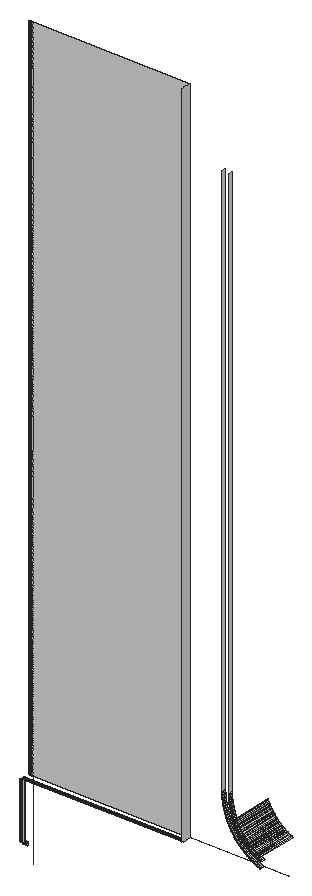
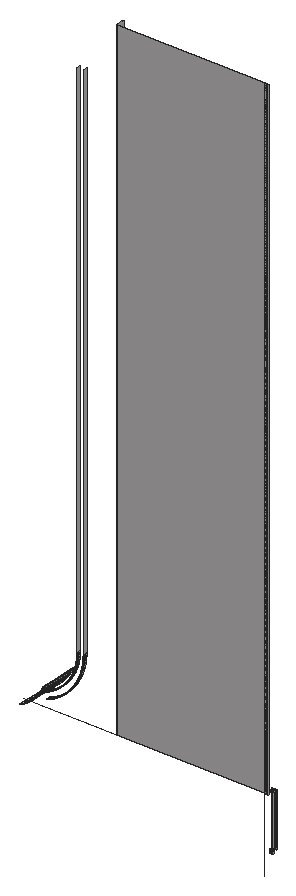
# SketchUp Ruby script. Lengths in inches.
U = 1.inch
M = Sketchup.active_model
def pt(a) = Geom::Point3d.new(a.map { |v| v * U })
def face(e, loops, mat)
  f = e.add_face(loops[0].map { |a| pt(a) })
  loops[1..].each { |l| e.add_face(l.map { |a| pt(a) }).erase! }
  f.material = f.back_material = mat if mat
  f
end
# faces: each face lists its corners as indices into pts; further lists are holes
def faces(e, pts, list, mat = nil) = list.each { |f| face(e, (f[0].is_a?(Array) ? f : [f]).map { |l| l.map { |i| pts[i] } }, mat) }
# xy, xz, yz: faces in a plane at the given z, y or x. An outline is a flat list of corners, or four numbers for a rectangle; further outlines are holes
def ring(l) = l.size == 4 ? [[l[0], l[1]], [l[2], l[1]], [l[2], l[3]], [l[0], l[3]]] : l.each_slice(2).to_a
def flat(e, list, mat, &to3) = list.each { |f| face(e, (f[0].is_a?(Array) ? f : [f]).map { |l| ring(l).map { |u, v| to3.(u, v) } }, mat) }
def xy(e, z, list, mat = nil) = flat(e, list, mat) { |x, y| [x, y, z] }
def xz(e, y, list, mat = nil) = flat(e, list, mat) { |x, z| [x, y, z] }
def yz(e, x, list, mat = nil) = flat(e, list, mat) { |y, z| [x, y, z] }
def lines(e, pts, list) = list.each { |a, b| e.add_line(pt(pts[a]), pt(pts[b])) }
# prism: a flat outline (further loops are holes) pulled along v
def prism(e, loops, v, mat = nil)
  f = face(e, loops, mat); d = Geom::Vector3d.new(v.map { |x| x * U })
  f.pushpull(f.normal.samedirection?(d) ? d.length : -d.length)
end
def box(e, o, s, mat = nil) = prism(e, [[o, [o[0] + s[0], o[1], o[2]], [o[0] + s[0], o[1] + s[1], o[2]], [o[0], o[1] + s[1], o[2]]]], [0, 0, s[2]], mat)
def at(x, y, z, deg = 0) = Geom::Transformation.translation(pt([x, y, z])) * Geom::Transformation.rotation(ORIGIN, Z_AXIS, deg.degrees)
def axes(o, x, y, z) = Geom::Transformation.new([*x, 0, *y, 0, *z, 0, *pt(o).to_a, 1])
def part(name) = M.definitions.add(name)
# library, detail: a bought-in or finely detailed component or shape, given as its bounding box
def library(name, o, s) = part(name).tap { |d| box(d.entities, o, s) }
def detail(e, o, s) = box(e.add_group.entities, o, s)
def put(e, d, t, mat = nil) = e.add_instance(d, t).tap { |i| i.material = mat if mat }
def group(e, t, mat = nil) = e.add_group.tap { |g| g.transformation = t; g.material = mat if mat }.entities
root = M.entities
M.materials.add("[Quartz Light Brown]").color = [215, 212, 212]
xz(root,143,[[215.8,133,216,150]],"[Quartz Light Brown]")
xz(root,143.01,[[215.41,133,215.61,150]],"[Quartz Light Brown]")
xz(root,143.75,[[215.625,149.75,215.8125,150],[215.8125,149.75,216,150],[216,149.75,263.5,150]],"[Quartz Light Brown]")
xz(root,144,[[215.63,132,215.82,133],[215.82,132,216,133]],"[Quartz Light Brown]")
xz(root,144.25,[[215.64,149.75,215.82,150],[215.82,149.75,216,150],[216,149.75,263.5,150]],"[Quartz Light Brown]")
xz(root,146,[[215.6875,150,215.84,354],[215.84,150,216,354],[216,150,263.5,354]],"[Quartz Light Brown]")
yz(root,263.5,[[143.75,149.75,143.75,150,143,150,143,354,143.75,354,143.75,354.25,144.25,354.25,144.25,354,146,354,146,150,144.25,150,144.25,149.75]],"[Quartz Light Brown]")
yz(root,275.5,[[143,167.76,144.25,168],[143,168,144.25,336]],"[Quartz Light Brown]")
yz(root,275.51,[[143,167.29,144.25,167.53]],"[Quartz Light Brown]")
yz(root,277.5,[[143,167.79,144.25,168],[143,168,144.25,336]],"[Quartz Light Brown]")
yz(root,277.51,[[143,167.37,144.25,167.58]],"[Quartz Light Brown]")
p = [[214.72,144.06,133],[214.72,144.06,132],[214.9,144.04,132],[214.9,144.04,133],[215.08,144.03,132],[215.08,144.03,133],
  [215.27,144.02,132],[215.27,144.02,133],[215.45,144.01,132],[215.45,144.01,133],[215.63,144,132],[215.63,144,133],
  [214.54,144.08,133],[214.54,144.08,132],[214.82,143.05,133],[214.82,143.05,150],[214.63,143.0625,150],[214.63,143.0625,133],
  [215.02,143.03,133],[215.02,143.03,150],[215.21,143.02,133],[215.21,143.02,150],[215.41,143.01,133],[215.41,143.01,150],
  [215.8,143,133],[215.8,143,150],[215.61,143.01,150],[215.61,143.01,133],[214.43,143.08,150],[214.43,143.08,133],
  [214.51,143.83,150],[214.7,143.81,150],[214.7,143.81,149.75],[214.51,143.83,149.75],[214.88,143.79,150],[214.88,143.79,149.75],
  [215.07,143.78,150],[215.07,143.78,149.75],[215.25,143.77,150],[215.25,143.77,149.75],[215.44,143.76,150],[215.44,143.76,149.75],
  [215.625,143.75,150],[215.625,143.75,149.75],[214.74,144.31,150],[214.5625,144.33,150],[214.5625,144.33,149.75],[214.74,144.31,149.75],
  [214.92,144.29,150],[214.92,144.29,149.75],[215.1,144.28,150],[215.1,144.28,149.75],[215.28,144.27,150],[215.28,144.27,149.75],
  [215.46,144.26,150],[215.46,144.26,149.75],[215.64,144.25,150],[215.64,144.25,149.75],[215.06,146.04,150],[215.06,146.04,354],
  [214.9,146.05,354],[214.9,146.05,150],[215.22,146.03,150],[215.22,146.03,354],[215.37,146.02,150],[215.37,146.02,354],
  [215.53,146.01,150],[215.53,146.01,354],[215.6875,146,150],[215.6875,146,354],[214.75,146.07,150],[214.75,146.07,354],
  [214.59,146.08,354],[214.59,146.08,150],[287.05,144.25,151.2],[287.05,143,151.2],[287.27,143,151.11],[287.27,144.25,151.11],
  [286.83,144.25,151.28],[286.83,143,151.28],[286.61,144.25,151.37],[286.61,143,151.37],[286.39,144.25,151.46],[286.39,143,151.46],
  [286.18,144.25,151.56],[286.18,143,151.56],[285.96,144.25,151.65],[285.96,143,151.65],[285.75,144.25,151.75],[285.75,143,151.75],
  [285.54,144.25,151.86],[285.54,143,151.86],[285.33,144.25,151.96],[285.33,143,151.96],[285.12,144.25,152.07],[285.12,143,152.07],
  [284.91,144.25,152.18],[284.91,143,152.18],[284.7,144.25,152.3],[284.7,143,152.3],[284.5,144.25,152.41],[284.5,143,152.41],
  [284.3,144.25,152.53],[284.3,143,152.53],[284.1,144.25,152.65],[284.1,143,152.65],[283.89,144.25,152.78],[283.89,143,152.78],
  [283.7,144.25,152.9],[283.7,143,152.9],[283.5,144.25,153.03],[283.5,143,153.03],[283.3,144.25,153.17],[283.3,143,153.17],
  [283.11,144.25,153.3],[283.11,143,153.3],[287.38,143,153.22],[287.18,143,153.3],[287.18,144.25,153.3],[287.38,144.25,153.22],
  [282.92,144.25,153.4375],[282.92,143,153.4375],[286.99,143,153.38],[286.99,144.25,153.38],[282.73,144.25,153.58],[282.73,143,153.58],
  [286.8,143,153.47],[286.8,144.25,153.47],[286.61,143,153.56],[286.61,144.25,153.56],[282.54,144.25,153.72],[282.54,143,153.72],
  [286.42,143,153.65],[286.42,144.25,153.65],[282.36,144.25,153.86],[282.36,143,153.86],[286.24,143,153.74],[286.05,143,153.84],
  [286.05,144.25,153.84],[286.24,144.25,153.74],[285.87,143,153.9375],[285.87,144.25,153.9375],[282.17,144.25,154.01],[282.17,143,154.01],
  [285.68,143,154.04],[285.68,144.25,154.04],[281.99,144.25,154.16],[281.99,143,154.16],[285.5,143,154.14],[285.5,144.25,154.14],
  [285.32,143,154.25],[285.32,144.25,154.25],[281.81,144.25,154.3125],[281.81,143,154.3125],[285.14,143,154.36],[285.14,144.25,154.36],
  [281.63,144.25,154.47],[281.63,143,154.47],[284.96,143,154.47],[284.96,144.25,154.47],[287.04,143,154.46],[287.22,143,154.38],
  [287.22,155,154.38],[287.04,155,154.46],[281.46,144.25,154.625],[281.46,143,154.625],[284.79,143,154.58],[284.79,144.25,154.58],
  [286.69,143,154.63],[286.87,143,154.55],[286.87,155,154.55],[286.69,155,154.63],[281.28,144.25,154.78],[281.28,143,154.78],
  [284.61,143,154.7],[284.61,144.25,154.7],[286.52,143,154.73],[286.52,155,154.73],[284.4375,143,154.8125],[284.4375,144.25,154.8125],
  [286.34,143,154.82],[286.34,155,154.82],[281.11,144.25,154.94],[281.11,143,154.94],[284.27,143,154.93],[284.27,144.25,154.93],
  [286.17,143,154.91],[286.17,155,154.91],[280.94,144.25,155.11],[280.94,143,155.11],[284.1,143,155.06],[284.1,144.25,155.06],
  [286,143,155.01],[286,155,155.01],[285.83,143,155.11],[285.83,155,155.11],[280.77,144.25,155.27],[280.77,143,155.27],
  [283.93,143,155.18],[283.93,144.25,155.18],[285.66,143,155.21],[285.66,155,155.21],[283.76,143,155.31],[283.76,144.25,155.31],
  [285.5,143,155.3125],[285.5,155,155.3125],[280.61,144.25,155.44],[280.61,143,155.44],[283.59,143,155.43],[283.59,144.25,155.43],
  [285.33,143,155.42],[285.33,155,155.42],[280.44,144.25,155.61],[280.44,143,155.61],[283.43,143,155.57],[283.43,144.25,155.57],
  [285.17,143,155.53],[285.17,155,155.53],[285,143,155.64],[285,155,155.64],[280.28,144.25,155.78],[280.28,143,155.78],
  [283.27,143,155.7],[283.27,144.25,155.7],[284.84,143,155.75],[284.84,155,155.75],[283.11,143,155.83],[283.11,144.25,155.83],
  [280.125,144.25,155.96],[280.125,143,155.96],[282.95,143,155.97],[282.95,144.25,155.97],[284.68,143,155.86],[284.68,155,155.86],
  [284.53,143,155.98],[284.53,155,155.98],[279.97,144.25,156.13],[279.97,143,156.13],[282.79,143,156.11],[282.79,144.25,156.11],
  [284.37,143,156.1],[284.37,155,156.1],[279.8125,144.25,156.31],[279.8125,143,156.31],[282.64,143,156.25],[282.64,144.25,156.25],
  [284.21,143,156.22],[284.21,155,156.22],[284.06,143,156.34],[284.06,155,156.34],[279.66,144.25,156.49],[279.66,143,156.49],
  [282.49,143,156.39],[282.49,144.25,156.39],[283.91,143,156.47],[283.91,155,156.47],[282.34,143,156.54],[282.34,144.25,156.54],
  [279.51,144.25,156.67],[279.51,143,156.67],[282.1875,143,156.6875],[282.1875,144.25,156.6875],[283.76,143,156.59],[283.76,155,156.59],
  [283.61,143,156.72],[283.61,155,156.72],[279.36,144.25,156.86],[279.36,143,156.86],[282.04,143,156.84],[282.04,144.25,156.84],
  [283.46,143,156.85],[283.46,155,156.85],[281.89,143,156.99],[281.89,144.25,156.99],[279.22,144.25,157.04],[279.22,143,157.04],
  [283.32,143,156.99],[283.32,155,156.99],[279.08,144.25,157.23],[279.08,143,157.23],[281.75,143,157.14],[281.75,144.25,157.14],
  [283.17,143,157.12],[283.17,155,157.12],[281.61,143,157.29],[281.61,144.25,157.29],[283.03,143,157.26],[283.03,155,157.26],
  [278.9375,144.25,157.42],[278.9375,143,157.42],[281.47,143,157.45],[281.47,144.25,157.45],[282.89,143,157.39],[282.89,155,157.39],
  [278.8,144.25,157.61],[278.8,143,157.61],[282.76,143,157.53],[282.76,155,157.53],[281.33,143,157.61],[281.33,144.25,157.61],
  [282.62,143,157.67],[282.62,155,157.67],[278.67,144.25,157.8],[278.67,143,157.8],[281.2,143,157.77],[281.2,144.25,157.77],
  [282.49,143,157.82],[282.49,155,157.82],[278.53,144.25,158],[278.53,143,158],[281.07,143,157.93],[281.07,144.25,157.93],
  [282.35,143,157.96],[282.35,155,157.96],[280.93,143,158.09],[280.93,144.25,158.09],[278.4,144.25,158.2],[278.4,143,158.2],
  [282.22,143,158.11],[282.22,155,158.11],[280.81,143,158.26],[280.81,144.25,158.26],[282.09,143,158.26],[282.09,155,158.26],
  [278.28,144.25,158.39],[278.28,143,158.39],[280.68,143,158.43],[280.68,144.25,158.43],[281.97,143,158.41],[281.97,155,158.41],
  [278.15,144.25,158.6],[278.15,143,158.6],[280.56,143,158.6],[280.56,144.25,158.6],[281.84,143,158.56],[281.84,155,158.56],
  [278.03,144.25,158.8],[278.03,143,158.8],[280.43,143,158.77],[280.43,144.25,158.77],[281.72,143,158.71],[281.72,155,158.71],
  [281.6,143,158.87],[281.6,155,158.87],[277.91,144.25,159],[277.91,143,159],[280.3125,143,158.9375],[280.3125,144.25,158.9375],
  [280.2,143,159.11],[280.2,144.25,159.11],[281.48,143,159.03],[281.48,155,159.03],[277.8,144.25,159.2],[277.8,143,159.2],
  [281.36,143,159.18],[281.36,155,159.18],[280.08,143,159.29],[280.08,144.25,159.29],[277.68,144.25,159.41],[277.68,143,159.41],
  [281.25,143,159.34],[281.25,155,159.34],[279.97,143,159.46],[279.97,144.25,159.46],[281.14,143,159.5],[281.14,155,159.5],
  [277.57,144.25,159.62],[277.57,143,159.62],[279.86,143,159.64],[279.86,144.25,159.64],[281.03,143,159.67],[281.03,155,159.67],
  [277.46,144.25,159.83],[277.46,143,159.83],[279.75,143,159.82],[279.75,144.25,159.82],[280.92,143,159.83],[280.92,155,159.83],
  [277.36,144.25,160.04],[277.36,143,160.04],[279.64,143,160],[279.64,144.25,160],[280.8125,143,160],[280.8125,155,160],
  [277.25,144.25,160.25],[277.25,143,160.25],[279.54,143,160.18],[279.54,144.25,160.18],[280.71,143,160.16],[280.71,155,160.16],
  [279.4375,143,160.37],[279.4375,144.25,160.37],[280.61,143,160.33],[280.61,155,160.33],[277.15,144.25,160.46],[277.15,143,160.46],
  [280.51,143,160.5],[280.51,155,160.5],[279.34,143,160.55],[279.34,144.25,160.55],[277.06,144.25,160.68],[277.06,143,160.68],
  [280.41,143,160.67],[280.41,155,160.67],[279.24,143,160.74],[279.24,144.25,160.74],[276.96,144.25,160.89],[276.96,143,160.89],
  [279.15,143,160.92],[279.15,144.25,160.92],[280.32,143,160.84],[280.32,155,160.84],[280.23,143,161.02],[280.23,155,161.02],
  [276.87,144.25,161.11],[276.87,143,161.11],[279.06,143,161.11],[279.06,144.25,161.11],[280.13,143,161.19],[280.13,155,161.19],
  [276.78,144.25,161.33],[276.78,143,161.33],[278.97,143,161.3],[278.97,144.25,161.3],[280.05,143,161.37],[280.05,155,161.37],
  [276.7,144.25,161.55],[276.7,143,161.55],[278.88,143,161.49],[278.88,144.25,161.49],[279.96,143,161.54],[279.96,155,161.54],
  [276.61,144.25,161.77],[276.61,143,161.77],[278.8,143,161.68],[278.8,144.25,161.68],[279.88,143,161.72],[279.88,155,161.72],
  [278.72,143,161.88],[278.72,144.25,161.88],[279.8,143,161.9],[279.8,155,161.9],[276.53,144.25,161.99],[276.53,143,161.99],
  [278.64,143,162.07],[278.64,144.25,162.07],[279.72,143,162.08],[279.72,155,162.08],[276.46,144.25,162.21],[276.46,143,162.21],
  [278.5625,143,162.27],[278.5625,144.25,162.27],[276.38,144.25,162.4375],[276.38,143,162.4375],[278.49,143,162.46],[278.49,144.25,162.46],
  [276.31,144.25,162.66],[276.31,143,162.66],[278.42,143,162.66],[278.42,144.25,162.66],[276.24,144.25,162.89],[276.24,143,162.89],
  [278.35,143,162.86],[278.35,144.25,162.86],[276.18,144.25,163.11],[276.18,143,163.11],[278.28,143,163.06],[278.28,144.25,163.06],
  [276.11,144.25,163.34],[276.11,143,163.34],[278.22,143,163.26],[278.22,144.25,163.26],[276.05,144.25,163.57],[276.05,143,163.57],
  [278.16,143,163.46],[278.16,144.25,163.46],[278.1,143,163.66],[278.1,144.25,163.66],[276,144.25,163.8],[276,143,163.8],
  [278.05,143,163.86],[278.05,144.25,163.86],[275.94,144.25,164.03],[275.94,143,164.03],[277.99,143,164.0625],[277.99,144.25,164.0625],
  [275.89,144.25,164.26],[275.89,143,164.26],[277.94,143,164.26],[277.94,144.25,164.26],[275.85,144.25,164.49],[275.85,143,164.49],
  [277.89,143,164.47],[277.89,144.25,164.47],[275.8,144.25,164.72],[275.8,143,164.72],[277.85,143,164.67],[277.85,144.25,164.67],
  [275.76,144.25,164.95],[275.76,143,164.95],[277.81,143,164.88],[277.81,144.25,164.88],[277.77,143,165.08],[277.77,144.25,165.08],
  [275.72,144.25,165.18],[275.72,143,165.18],[277.73,143,165.29],[277.73,144.25,165.29],[275.6875,144.25,165.42],[275.6875,143,165.42],
  [277.7,143,165.5],[277.7,144.25,165.5],[275.65,144.25,165.65],[275.65,143,165.65],[277.67,143,165.7],[277.67,144.25,165.7],
  [275.625,144.25,165.88],[275.625,143,165.88],[277.64,143,165.91],[277.64,144.25,165.91],[275.6,144.25,166.12],[275.6,143,166.12],
  [277.61,143,166.12],[277.61,144.25,166.12],[275.58,144.25,166.35],[275.58,143,166.35],[277.59,143,166.33],[277.59,144.25,166.33],
  [277.57,143,166.54],[277.57,144.25,166.54],[275.56,144.25,166.59],[275.56,143,166.59],[277.55,143,166.74],[277.55,144.25,166.74],
  [275.54,144.25,166.82],[275.54,143,166.82],[277.53,143,166.95],[277.53,144.25,166.95],[275.52,144.25,167.06],[275.52,143,167.06],
  [277.52,143,167.16],[277.52,144.25,167.16],[275.51,144.25,167.29],[275.51,143,167.29],[277.51,143,167.37],[277.51,144.25,167.37],
  [275.5,144.25,167.76],[275.5,143,167.76],[275.51,143,167.53],[275.51,144.25,167.53],[277.51,143,167.58],[277.5,143,167.79],
  [277.5,144.25,167.79],[277.51,144.25,167.58],[216,146,150],[216,146,126],[263.5,146,150],[293.5,146,150]]
faces(root,p,[[0,1,2,3],[3,2,4,5],[5,4,6,7],[7,6,8,9],[9,8,10,11],[12,13,1,0],[14,15,16,17],[18,19,15,14],
  [20,21,19,18],[22,23,21,20],[24,25,26,27],[17,16,28,29],[30,31,32,33],[31,34,35,32],[34,36,37,35],[36,38,39,37],
  [38,40,41,39],[40,42,43,41],[44,45,46,47],[48,44,47,49],[50,48,49,51],[52,50,51,53],[54,52,53,55],[56,54,55,57],
  [58,59,60,61],[62,63,59,58],[64,65,63,62],[66,67,65,64],[68,69,67,66],[70,71,72,73],[61,60,71,70],[74,75,76,77],
  [78,79,75,74],[80,81,79,78],[82,83,81,80],[84,85,83,82],[86,87,85,84],[88,89,87,86],[90,91,89,88],[92,93,91,90],
  [94,95,93,92],[96,97,95,94],[98,99,97,96],[100,101,99,98],[102,103,101,100],[104,105,103,102],[106,107,105,104],[108,109,107,106],
  [110,111,109,108],[112,113,111,110],[114,115,113,112],[116,117,118,119],[120,121,115,114],[117,122,123,118],[124,125,121,120],[122,126,127,123],
  [126,128,129,127],[130,131,125,124],[128,132,133,129],[134,135,131,130],[136,137,138,139],[132,136,139,133],[137,140,141,138],[142,143,135,134],
  [140,144,145,141],[146,147,143,142],[144,148,149,145],[148,150,151,149],[152,153,147,146],[150,154,155,151],[156,157,153,152],[154,158,159,155],
  [160,161,162,163],[164,165,157,156],[158,166,167,159],[168,169,170,171],[169,160,163,170],[172,173,165,164],[166,174,175,167],[176,168,171,177],
  [174,178,179,175],[180,176,177,181],[182,183,173,172],[178,184,185,179],[186,180,181,187],[188,189,183,182],[184,190,191,185],[192,186,187,193],
  [194,192,193,195],[196,197,189,188],[190,198,199,191],[200,194,195,201],[198,202,203,199],[204,200,201,205],[206,207,197,196],[202,208,209,203],
  [210,204,205,211],[212,213,207,206],[208,214,215,209],[216,210,211,217],[218,216,217,219],[220,221,213,212],[214,222,223,215],[224,218,219,225],
  [222,226,227,223],[228,229,221,220],[226,230,231,227],[232,224,225,233],[234,232,233,235],[236,237,229,228],[230,238,239,231],[240,234,235,241],
  [242,243,237,236],[238,244,245,239],[246,240,241,247],[248,246,247,249],[250,251,243,242],[244,252,253,245],[254,248,249,255],[252,256,257,253],
  [258,259,251,250],[256,260,261,257],[262,254,255,263],[264,262,263,265],[266,267,259,258],[260,268,269,261],[270,264,265,271],[268,272,273,269],
  [274,275,267,266],[276,270,271,277],[278,279,275,274],[272,280,281,273],[282,276,277,283],[280,284,285,281],[286,282,283,287],[288,289,279,278],
  [284,290,291,285],[292,286,287,293],[294,295,289,288],[296,292,293,297],[290,298,299,291],[300,296,297,301],[302,303,295,294],[298,304,305,299],
  [306,300,301,307],[308,309,303,302],[304,310,311,305],[312,306,307,313],[310,314,315,311],[316,317,309,308],[318,312,313,319],[314,320,321,315],
  [322,318,319,323],[324,325,317,316],[320,326,327,321],[328,322,323,329],[330,331,325,324],[326,332,333,327],[334,328,329,335],[336,337,331,330],
  [332,338,339,333],[340,334,335,341],[342,340,341,343],[344,345,337,336],[338,346,347,339],[346,348,349,347],[350,342,343,351],[352,353,345,344],
  [354,350,351,355],[348,356,357,349],[358,359,353,352],[360,354,355,361],[356,362,363,357],[364,360,361,365],[366,367,359,358],[362,368,369,363],
  [370,364,365,371],[372,373,367,366],[368,374,375,369],[376,370,371,377],[378,379,373,372],[374,380,381,375],[382,376,377,383],[384,385,379,378],
  [380,386,387,381],[388,382,383,389],[386,390,391,387],[392,388,389,393],[394,395,385,384],[396,392,393,397],[390,398,399,391],[400,401,395,394],
  [402,396,397,403],[398,404,405,399],[406,407,401,400],[404,408,409,405],[410,402,403,411],[412,410,411,413],[414,415,407,406],[408,416,417,409],
  [418,412,413,419],[420,421,415,414],[416,422,423,417],[424,418,419,425],[426,427,421,420],[422,428,429,423],[430,424,425,431],[432,433,427,426],
  [428,434,435,429],[436,430,431,437],[434,438,439,435],[440,436,437,441],[442,443,433,432],[438,444,445,439],[446,440,441,447],[448,449,443,442],
  [444,450,451,445],[452,453,449,448],[450,454,455,451],[456,457,453,452],[454,458,459,455],[460,461,457,456],[458,462,463,459],[464,465,461,460],
  [462,466,467,463],[468,469,465,464],[466,470,471,467],[472,473,469,468],[470,474,475,471],[474,476,477,475],[478,479,473,472],[476,480,481,477],
  [482,483,479,478],[480,484,485,481],[486,487,483,482],[484,488,489,485],[490,491,487,486],[488,492,493,489],[494,495,491,490],[492,496,497,493],
  [498,499,495,494],[496,500,501,497],[500,502,503,501],[504,505,499,498],[502,506,507,503],[508,509,505,504],[506,510,511,507],[512,513,509,508],
  [510,514,515,511],[516,517,513,512],[514,518,519,515],[520,521,517,516],[518,522,523,519],[524,525,521,520],[522,526,527,523],[526,528,529,527],
  [530,531,525,524],[528,532,533,529],[534,535,531,530],[532,536,537,533],[538,539,535,534],[536,540,541,537],[542,543,539,538],[540,544,545,541],
  [546,547,548,549],[550,551,552,553]],"[Quartz Light Brown]")
lines(root,p,[[554,555],[556,557]])
